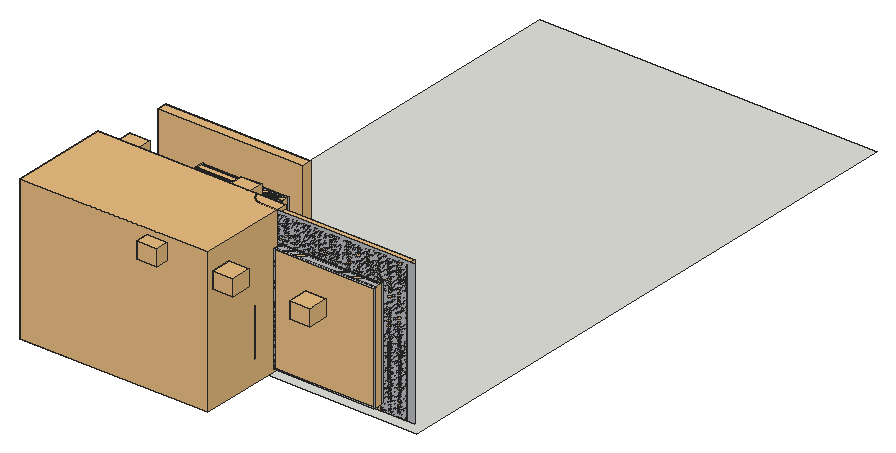
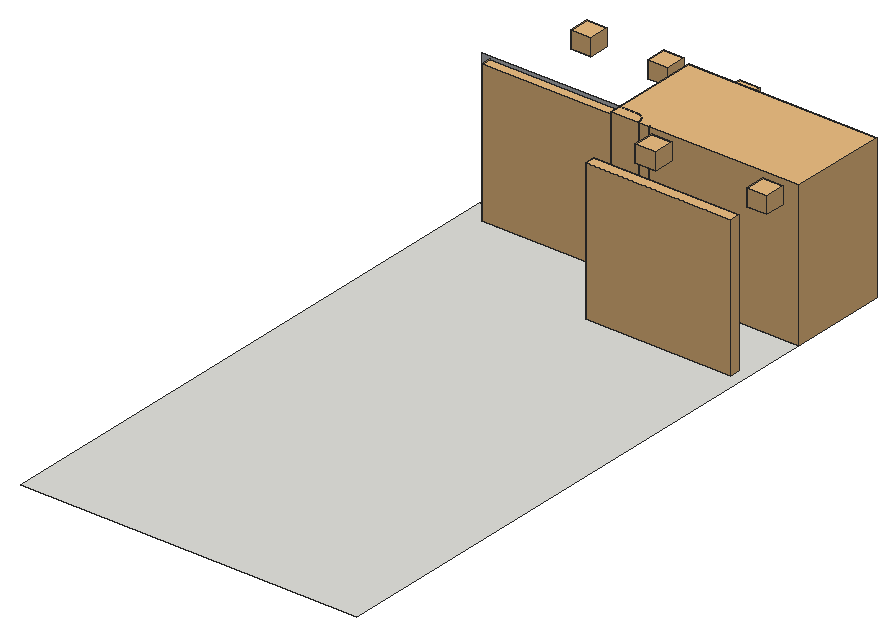
# SketchUp Ruby script. Lengths in inches.
U = 1.inch
M = Sketchup.active_model
def pt(a) = Geom::Point3d.new(a.map { |v| v * U })
def face(e, loops, mat)
  f = e.add_face(loops[0].map { |a| pt(a) })
  loops[1..].each { |l| e.add_face(l.map { |a| pt(a) }).erase! }
  f.material = f.back_material = mat if mat
  f
end
# faces: each face lists its corners as indices into pts; further lists are holes
def faces(e, pts, list, mat = nil) = list.each { |f| face(e, (f[0].is_a?(Array) ? f : [f]).map { |l| l.map { |i| pts[i] } }, mat) }
# xy, xz, yz: faces in a plane at the given z, y or x. An outline is a flat list of corners, or four numbers for a rectangle; further outlines are holes
def ring(l) = l.size == 4 ? [[l[0], l[1]], [l[2], l[1]], [l[2], l[3]], [l[0], l[3]]] : l.each_slice(2).to_a
def flat(e, list, mat, &to3) = list.each { |f| face(e, (f[0].is_a?(Array) ? f : [f]).map { |l| ring(l).map { |u, v| to3.(u, v) } }, mat) }
def xy(e, z, list, mat = nil) = flat(e, list, mat) { |x, y| [x, y, z] }
def xz(e, y, list, mat = nil) = flat(e, list, mat) { |x, z| [x, y, z] }
def yz(e, x, list, mat = nil) = flat(e, list, mat) { |y, z| [x, y, z] }
def lines(e, pts, list) = list.each { |a, b| e.add_line(pt(pts[a]), pt(pts[b])) }
# prism: a flat outline (further loops are holes) pulled along v
def prism(e, loops, v, mat = nil)
  f = face(e, loops, mat); d = Geom::Vector3d.new(v.map { |x| x * U })
  f.pushpull(f.normal.samedirection?(d) ? d.length : -d.length)
end
def box(e, o, s, mat = nil) = prism(e, [[o, [o[0] + s[0], o[1], o[2]], [o[0] + s[0], o[1] + s[1], o[2]], [o[0], o[1] + s[1], o[2]]]], [0, 0, s[2]], mat)
def at(x, y, z, deg = 0) = Geom::Transformation.translation(pt([x, y, z])) * Geom::Transformation.rotation(ORIGIN, Z_AXIS, deg.degrees)
def axes(o, x, y, z) = Geom::Transformation.new([*x, 0, *y, 0, *z, 0, *pt(o).to_a, 1])
def part(name) = M.definitions.add(name)
# library, detail: a bought-in or finely detailed component or shape, given as its bounding box
def library(name, o, s) = part(name).tap { |d| box(d.entities, o, s) }
def detail(e, o, s) = box(e.add_group.entities, o, s)
def put(e, d, t, mat = nil) = e.add_instance(d, t).tap { |i| i.material = mat if mat }
def group(e, t, mat = nil) = e.add_group.tap { |g| g.transformation = t; g.material = mat if mat }.entities
root = M.entities
M.materials.add("1427 AP 686 ARMOUR-N").color = [184, 186, 189]
c1 = library("Untitled",[0,0,0],[96,5.09,80])
c2 = library("Curtains",[0,0,0],[121.73,8.19,117.22])
c3 = library("Group\#9",[-1,-1,0],[157,81.05,120])
c4 = library("2",[-6.43,-6.43,-13.78],[16.84,16.84,13.78])
xy(root,252,[[21,129.92,141,129.92,141.29,129.93,141.58,129.93,142.16,129.95,143.03,130.01,143.31,130.04,143.89,130.1,144.47,130.18,144.75,130.22,145.04,130.27,145.32,130.32,145.61,130.37,145.89,130.43,146.18,130.49,146.46,130.55,147.02,130.69,148.14,131.01,148.41,131.1,148.69,131.19,148.96,131.28,149.24,131.38,149.51,131.48,150.32,131.81,150.58,131.92,150.85,132.04,151.11,132.16,151.375,132.28,151.64,132.41,151.89,132.54,152.15,132.67,152.41,132.81,152.91,133.09,153.17,133.24,153.41,133.39,153.91,133.69,154.63,134.17,155.11,134.51,155.57,134.85,156.03,135.21,156.25,135.4,156.48,135.58,156.7,135.77,156.91,135.96,157.13,136.15,157.97,136.95,158.17,137.16,158.375,137.37,158.57,137.58,158.77,137.79,159.53,138.67,159.71,138.9,160.07,139.35,160.24,139.58,160.42,139.82,160.58,140.05,160.75,140.29,161.07,140.77,161.23,141.02,161.39,141.26,161.54,141.51,161.6875,141.76,161.83,142.01,162.11,142.51,162.25,142.77,162.64,143.55,162.76,143.8125,162.88,144.07,163.12,144.61,163.34,145.14,163.44,145.41,163.54,145.6875,163.64,145.96,163.73,146.23,163.82,146.51,163.91,146.78,164,147.0625,164.08,147.34,164.16,147.62,164.37,148.46,164.43,148.75,164.5,149.03,164.55,149.3125,164.61,149.6,164.66,149.88,164.7,150.17,164.75,150.46,164.79,150.74,164.82,151.03,164.86,151.32,164.89,151.61,164.91,151.9,164.9375,152.1875,164.96,152.48,164.97,152.76,165,153.63,165,192,290,192,290,672,9,672,9,141.61,9.01,141.45,9.02,141.3,9.04,140.98,9.05,140.83,9.07,140.67,9.08,140.51,9.1,140.36,9.125,140.2,9.15,140.05,9.17,139.89,9.2,139.74,9.23,139.58,9.26,139.43,9.3,139.28,9.33,139.125,9.37,138.97,9.49,138.52,9.64,138.07,9.6875,137.92,9.74,137.77,9.8,137.625,9.85,137.48,9.91,137.33,9.97,137.1875,10.04,137.04,10.1,136.9,10.45,136.2,10.53,136.0625,10.61,135.92,10.6875,135.79,10.77,135.65,10.85,135.52,10.9375,135.39,11.02,135.26,11.29,134.87,11.39,134.74,11.48,134.62,11.58,134.5,11.67,134.37,11.77,134.25,11.98,134.01,12.08,133.89,12.1875,133.78,12.3,133.66,12.4,133.55,12.51,133.4375,12.625,133.33,12.74,133.22,12.85,133.11,12.97,133.01,13.09,132.9,13.69,132.4,13.95,132.22,14.07,132.125,14.2,132.03,14.33,131.95,14.46,131.86,14.6,131.78,14.73,131.69,14.86,131.61,15.14,131.45,15.27,131.38,15.41,131.3,15.83,131.09,15.98,131.03,16.12,130.96,16.26,130.9,16.41,130.84,16.55,130.78,16.7,130.72,16.85,130.67,16.99,130.61,17.14,130.5625,17.29,130.51,17.44,130.46,17.59,130.42,17.89,130.33,18.05,130.29,18.2,130.26,18.35,130.22,18.51,130.1875,18.66,130.15,18.8125,130.125,18.97,130.1,19.12,130.07,19.28,130.05,19.43,130.03,19.75,129.99,19.9,129.97,20.22,129.95,20.37,129.94,20.53,129.93,20.84,129.93]])
xy(root,258,[[170,192,254,201]],"1427 AP 686 ARMOUR-N")
xy(root,342,[[56,252,128,261]],"1427 AP 686 ARMOUR-N")
xy(root,348,[[170,192,254,201]],"1427 AP 686 ARMOUR-N")
xz(root,201,[[151.78,252,151.89,372],[[151.89,252,281,372],[170,258,254,348]]],"1427 AP 686 ARMOUR-N")
xz(root,201.01,[[151.57,252,151.67,372]],"1427 AP 686 ARMOUR-N")
xz(root,201.02,[[151.35,252,151.46,372]],"1427 AP 686 ARMOUR-N")
yz(root,56,[[252,252,261,342]],"1427 AP 686 ARMOUR-N")
yz(root,128,[[252,252,261,342]],"1427 AP 686 ARMOUR-N")
yz(root,134,[[209.78,252,210,372]],"1427 AP 686 ARMOUR-N")
yz(root,134.01,[[209.35,252,209.57,372]],"1427 AP 686 ARMOUR-N")
yz(root,143,[[209.78,252,209.89,372]],"1427 AP 686 ARMOUR-N")
yz(root,143.01,[[209.57,252,209.67,372]],"1427 AP 686 ARMOUR-N")
yz(root,143.02,[[209.35,252,209.46,372]],"1427 AP 686 ARMOUR-N")
yz(root,170,[[192,258,201,348]],"1427 AP 686 ARMOUR-N")
yz(root,254,[[192,258,201,348]],"1427 AP 686 ARMOUR-N")
p = [[151.02,201.05,372],[151.13,201.04,372],[151.13,201.04,252],[151.02,201.05,252],[151.24,201.03,372],[151.24,201.03,252],
  [151.35,201.02,372],[151.35,201.02,252],[151.46,201.02,372],[151.57,201.01,372],[151.57,201.01,252],[151.46,201.02,252],
  [151.67,201.01,372],[151.78,201,372],[151.78,201,252],[151.67,201.01,252],[150.27,201.17,372],[150.38,201.15,372],
  [150.38,201.15,252],[150.27,201.17,252],[150.48,201.13,372],[150.48,201.13,252],[150.59,201.11,372],[150.59,201.11,252],
  [150.7,201.09,372],[150.7,201.09,252],[150.81,201.08,372],[150.81,201.08,252],[150.92,201.07,372],[150.92,201.07,252],
  [149.85,201.26,372],[149.95,201.24,372],[149.95,201.24,252],[149.85,201.26,252],[150.06,201.21,372],[150.06,201.21,252],
  [150.16,201.1875,372],[150.16,201.1875,252],[149.43,201.375,372],[149.53,201.35,372],[149.53,201.35,252],[149.43,201.375,252],
  [149.64,201.32,372],[149.64,201.32,252],[149.74,201.29,372],[149.74,201.29,252],[149.12,201.47,372],[149.22,201.44,372],
  [149.22,201.44,252],[149.12,201.47,252],[149.32,201.41,372],[149.32,201.41,252],[148.81,201.58,372],[148.91,201.55,372],
  [148.91,201.55,252],[148.81,201.58,252],[149.01,201.51,372],[149.01,201.51,252],[148.61,201.66,372],[148.71,201.625,372],
  [148.71,201.625,252],[148.61,201.66,252],[148.31,201.79,372],[148.41,201.75,372],[148.41,201.75,252],[148.31,201.79,252],
  [148.51,201.71,372],[148.51,201.71,252],[148.11,201.88,372],[148.21,201.84,372],[148.21,201.84,252],[148.11,201.88,252],
  [147.91,201.98,372],[148.01,201.93,372],[148.01,201.93,252],[147.91,201.98,252],[147.72,202.08,372],[147.82,202.03,372],
  [147.82,202.03,252],[147.72,202.08,252],[147.53,202.1875,372],[147.625,202.13,372],[147.625,202.13,252],[147.53,202.1875,252],
  [147.34,202.3,372],[147.4375,202.24,372],[147.4375,202.24,252],[147.34,202.3,252],[147.25,202.35,372],[147.25,202.35,252],
  [147.07,202.47,372],[147.16,202.41,372],[147.16,202.41,252],[147.07,202.47,252],[146.89,202.59,372],[146.98,202.53,372],
  [146.98,202.53,252],[146.89,202.59,252],[146.8,202.66,372],[146.8,202.66,252],[146.62,202.78,372],[146.71,202.72,372],
  [146.71,202.72,252],[146.62,202.78,252],[146.45,202.92,372],[146.54,202.85,372],[146.54,202.85,252],[146.45,202.92,252],
  [146.36,202.98,372],[146.36,202.98,252],[146.28,203.05,372],[146.28,203.05,252],[146.11,203.19,372],[146.2,203.12,372],
  [146.2,203.12,252],[146.11,203.19,252],[146.03,203.26,372],[146.03,203.26,252],[145.87,203.41,372],[145.95,203.34,372],
  [145.95,203.34,252],[145.87,203.41,252],[145.79,203.48,372],[145.79,203.48,252],[145.71,203.56,372],[145.71,203.56,252],
  [145.64,203.64,372],[145.64,203.64,252],[145.56,203.71,372],[145.56,203.71,252],[145.48,203.79,372],[145.48,203.79,252],
  [145.41,203.87,372],[145.41,203.87,252],[145.34,203.95,372],[145.34,203.95,252],[145.19,204.11,372],[145.26,204.03,372],
  [145.26,204.03,252],[145.19,204.11,252],[145.12,204.2,372],[145.12,204.2,252],[145.05,204.28,372],[145.05,204.28,252],
  [144.98,204.36,372],[144.98,204.36,252],[144.85,204.54,372],[144.92,204.45,372],[144.92,204.45,252],[144.85,204.54,252],
  [144.78,204.62,372],[144.78,204.62,252],[144.72,204.71,372],[144.72,204.71,252],[144.66,204.8,372],[144.66,204.8,252],
  [144.59,204.89,372],[144.59,204.89,252],[144.53,204.98,372],[144.53,204.98,252],[144.47,205.07,372],[144.47,205.07,252],
  [144.41,205.16,372],[144.41,205.16,252],[144.35,205.25,372],[144.35,205.25,252],[144.24,205.4375,372],[144.3,205.34,372],
  [144.3,205.34,252],[144.24,205.4375,252],[144.1875,205.53,372],[144.1875,205.53,252],[144.13,205.625,372],[144.13,205.625,252],
  [144.08,205.72,372],[144.08,205.72,252],[144.03,205.82,372],[144.03,205.82,252],[143.98,205.91,372],[143.98,205.91,252],
  [143.93,206.01,372],[143.93,206.01,252],[143.88,206.11,372],[143.88,206.11,252],[143.84,206.21,372],[143.84,206.21,252],
  [143.79,206.31,372],[143.79,206.31,252],[143.75,206.41,372],[143.75,206.41,252],[143.71,206.51,372],[143.71,206.51,252],
  [143.66,206.61,372],[143.66,206.61,252],[143.625,206.71,372],[143.625,206.71,252],[143.58,206.81,372],[143.58,206.81,252],
  [143.55,206.91,372],[143.55,206.91,252],[143.51,207.01,372],[143.51,207.01,252],[143.47,207.12,372],[143.47,207.12,252],
  [143.44,207.22,372],[143.44,207.22,252],[143.41,207.32,372],[143.41,207.32,252],[143.375,207.43,372],[143.375,207.43,252],
  [143.35,207.53,372],[143.35,207.53,252],[143.32,207.64,372],[143.32,207.64,252],[143.29,207.74,372],[143.29,207.74,252],
  [143.26,207.85,372],[143.26,207.85,252],[143.24,207.95,372],[143.24,207.95,252],[143.21,208.06,372],[143.21,208.06,252],
  [143.1875,208.16,372],[143.1875,208.16,252],[143.17,208.27,372],[143.17,208.27,252],[143.15,208.38,372],[143.15,208.38,252],
  [143.13,208.48,372],[143.13,208.48,252],[143.11,208.59,372],[143.11,208.59,252],[143.09,208.7,372],[143.09,208.7,252],
  [143.08,208.81,372],[143.08,208.81,252],[143.07,208.92,372],[143.07,208.92,252],[143.05,209.02,372],[143.05,209.02,252],
  [143.04,209.13,372],[143.04,209.13,252],[143.03,209.24,372],[143.03,209.24,252],[143.02,209.35,372],[143.02,209.35,252],
  [143.01,209.57,372],[143.02,209.46,372],[143.02,209.46,252],[143.01,209.57,252],[134.01,209.57,372],[134,209.78,372],
  [134,209.78,252],[134.01,209.57,252],[143,209.78,372],[143.01,209.67,372],[143.01,209.67,252],[143,209.78,252]]
faces(root,p,[[0,1,2,3],[1,4,5,2],[4,6,7,5],[8,9,10,11],[12,13,14,15],[16,17,18,19],[17,20,21,18],[20,22,23,21],
  [22,24,25,23],[24,26,27,25],[26,28,29,27],[28,0,3,29],[30,31,32,33],[31,34,35,32],[34,36,37,35],[36,16,19,37],
  [38,39,40,41],[39,42,43,40],[42,44,45,43],[44,30,33,45],[46,47,48,49],[47,50,51,48],[50,38,41,51],[52,53,54,55],
  [53,56,57,54],[56,46,49,57],[58,59,60,61],[59,52,55,60],[62,63,64,65],[63,66,67,64],[66,58,61,67],[68,69,70,71],
  [69,62,65,70],[72,73,74,75],[73,68,71,74],[76,77,78,79],[77,72,75,78],[80,81,82,83],[81,76,79,82],[84,85,86,87],
  [85,80,83,86],[88,84,87,89],[90,91,92,93],[91,88,89,92],[94,95,96,97],[95,90,93,96],[98,94,97,99],[100,101,102,103],
  [101,98,99,102],[104,105,106,107],[105,100,103,106],[108,104,107,109],[110,108,109,111],[112,113,114,115],[113,110,111,114],[116,112,115,117],
  [118,119,120,121],[119,116,117,120],[122,118,121,123],[124,122,123,125],[126,124,125,127],[128,126,127,129],[130,128,129,131],[132,130,131,133],
  [134,132,133,135],[136,137,138,139],[137,134,135,138],[140,136,139,141],[142,140,141,143],[144,142,143,145],[146,147,148,149],[147,144,145,148],
  [150,146,149,151],[152,150,151,153],[154,152,153,155],[156,154,155,157],[158,156,157,159],[160,158,159,161],[162,160,161,163],[164,162,163,165],
  [166,167,168,169],[167,164,165,168],[170,166,169,171],[172,170,171,173],[174,172,173,175],[176,174,175,177],[178,176,177,179],[180,178,179,181],
  [182,180,181,183],[184,182,183,185],[186,184,185,187],[188,186,187,189],[190,188,189,191],[192,190,191,193],[194,192,193,195],[196,194,195,197],
  [198,196,197,199],[200,198,199,201],[202,200,201,203],[204,202,203,205],[206,204,205,207],[208,206,207,209],[210,208,209,211],[212,210,211,213],
  [214,212,213,215],[216,214,215,217],[218,216,217,219],[220,218,219,221],[222,220,221,223],[224,222,223,225],[226,224,225,227],[228,226,227,229],
  [230,228,229,231],[232,230,231,233],[234,232,233,235],[236,234,235,237],[238,236,237,239],[240,238,239,241],[242,240,241,243],[244,242,243,245],
  [246,247,248,249],[250,251,252,253],[254,255,256,257]],"1427 AP 686 ARMOUR-N")
put(root,c1,axes([56,254,252],[0.75,0,0],[0,1,0],[0,0,1.125]),"1427 AP 686 ARMOUR-N")
put(root,c2,at(152.62,201,252),"1427 AP 686 ARMOUR-N")
put(root,c2,at(18,261,252),"1427 AP 686 ARMOUR-N")
put(root,c3,axes([165,129.92,252],[-1,0,0],[0,1,0],[0,0,1]),"1427 AP 686 ARMOUR-N")
put(root,c1,axes([170,194,258],[0.875,0,0],[0,1,0],[0,0,1.125]),"1427 AP 686 ARMOUR-N")
put(root,c4,at(249.01,124.51,367.38))
put(root,c4,at(185.14,124.51,367.38))
put(root,c4,at(121.26,124.51,367.38))
put(root,c4,at(121.26,170.76,367.38))
put(root,c4,at(121.26,217.01,367.38))
put(root,c4,at(28.01,217.01,367.38))
